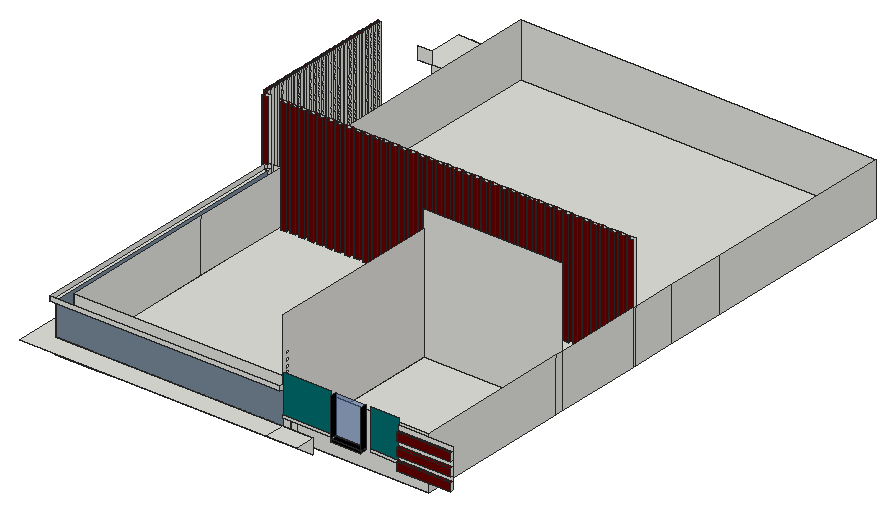
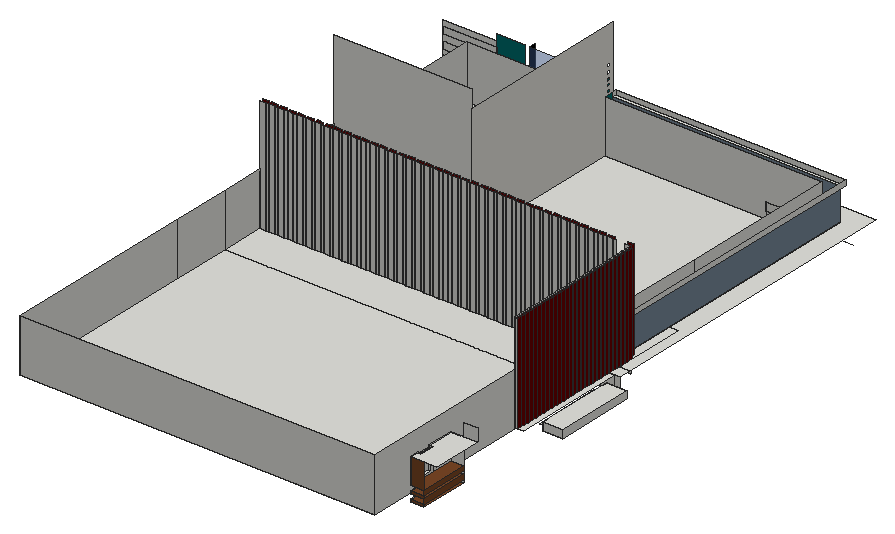
# SketchUp Ruby script. Lengths in inches.
U = 1.inch
M = Sketchup.active_model
def pt(a) = Geom::Point3d.new(a.map { |v| v * U })
def face(e, loops, mat)
  f = e.add_face(loops[0].map { |a| pt(a) })
  loops[1..].each { |l| e.add_face(l.map { |a| pt(a) }).erase! }
  f.material = f.back_material = mat if mat
  f
end
# faces: each face lists its corners as indices into pts; further lists are holes
def faces(e, pts, list, mat = nil) = list.each { |f| face(e, (f[0].is_a?(Array) ? f : [f]).map { |l| l.map { |i| pts[i] } }, mat) }
# xy, xz, yz: faces in a plane at the given z, y or x. An outline is a flat list of corners, or four numbers for a rectangle; further outlines are holes
def ring(l) = l.size == 4 ? [[l[0], l[1]], [l[2], l[1]], [l[2], l[3]], [l[0], l[3]]] : l.each_slice(2).to_a
def flat(e, list, mat, &to3) = list.each { |f| face(e, (f[0].is_a?(Array) ? f : [f]).map { |l| ring(l).map { |u, v| to3.(u, v) } }, mat) }
def xy(e, z, list, mat = nil) = flat(e, list, mat) { |x, y| [x, y, z] }
def xz(e, y, list, mat = nil) = flat(e, list, mat) { |x, z| [x, y, z] }
def yz(e, x, list, mat = nil) = flat(e, list, mat) { |y, z| [x, y, z] }
def lines(e, pts, list) = list.each { |a, b| e.add_line(pt(pts[a]), pt(pts[b])) }
# prism: a flat outline (further loops are holes) pulled along v
def prism(e, loops, v, mat = nil)
  f = face(e, loops, mat); d = Geom::Vector3d.new(v.map { |x| x * U })
  f.pushpull(f.normal.samedirection?(d) ? d.length : -d.length)
end
def box(e, o, s, mat = nil) = prism(e, [[o, [o[0] + s[0], o[1], o[2]], [o[0] + s[0], o[1] + s[1], o[2]], [o[0], o[1] + s[1], o[2]]]], [0, 0, s[2]], mat)
def at(x, y, z, deg = 0) = Geom::Transformation.translation(pt([x, y, z])) * Geom::Transformation.rotation(ORIGIN, Z_AXIS, deg.degrees)
def axes(o, x, y, z) = Geom::Transformation.new([*x, 0, *y, 0, *z, 0, *pt(o).to_a, 1])
def part(name) = M.definitions.add(name)
# library, detail: a bought-in or finely detailed component or shape, given as its bounding box
def library(name, o, s) = part(name).tap { |d| box(d.entities, o, s) }
def detail(e, o, s) = box(e.add_group.entities, o, s)
def put(e, d, t, mat = nil) = e.add_instance(d, t).tap { |i| i.material = mat if mat }
def group(e, t, mat = nil) = e.add_group.tap { |g| g.transformation = t; g.material = mat if mat }.entities
root = M.entities
M.materials.add("[0110_LightSlateGray]").color = [119, 136, 153]
M.materials.add("[Color A08]").color = [102, 0, 0]
M.materials.add("[Color H07]1").color = [0, 109, 109]
M.materials.add("[Color M09]").color = [0, 0, 0]
M.materials.add("[Marble Carrara Gold Floor Tile]").color = [225, 223, 217]
M.materials.add("[Translucent Glass Blue]1").color = [78, 117, 186]
M.materials["[Translucent Glass Blue]1"].alpha = 0.5
M.materials.add("[Wood Veneer 01]").color = [120, 70, 37]
xy(root,255.61,[[98.54,121.91,294.79,121.91,294.79,352.8,290.69,352.8,290.69,355.8,287.79,355.8,287.79,352.8,282.44,352.8,282.44,355.8,279.54,355.8,279.54,352.8,274.19,352.8,274.19,355.8,271.29,355.8,271.29,352.8,265.94,352.8,265.94,355.8,263.04,355.8,263.04,352.8,257.69,352.8,257.69,355.8,254.79,355.8,254.79,352.8,249.44,352.8,249.44,355.8,246.54,355.8,246.54,352.8,241.19,352.8,241.19,355.8,238.29,355.8,238.29,352.8,232.94,352.8,232.94,355.8,230.04,355.8,230.04,352.8,224.69,352.8,224.69,355.8,221.79,355.8,221.79,352.8,216.44,352.8,216.44,355.8,213.54,355.8,213.54,352.8,208.19,352.8,208.19,355.8,205.29,355.8,205.29,352.8,199.94,352.8,199.94,355.8,197.04,355.8,197.04,352.8,191.69,352.8,191.69,355.8,188.79,355.8,188.79,352.8,183.44,352.8,183.44,355.8,180.54,355.8,180.54,352.8,175.19,352.8,175.19,355.8,172.29,355.8,172.29,352.8,166.94,352.8,166.94,355.8,164.04,355.8,164.04,352.8,158.69,352.8,158.69,355.8,155.79,355.8,155.79,352.8,150.44,352.8,150.44,355.8,147.54,355.8,147.54,352.8,142.19,352.8,142.19,355.8,139.29,355.8,139.29,352.8,133.94,352.8,133.94,355.8,131.04,355.8,131.04,352.8,125.69,352.8,125.69,355.8,122.79,355.8,122.79,352.8,117.44,352.8,117.44,355.8,114.54,355.8,114.54,352.8,109.19,352.8,109.19,355.8,106.29,355.8,106.29,352.8,100.94,352.8,100.94,355.8,98.54,355.8],[294.79,121.91,419.79,272.1],[294.79,272.1,419.79,272.1,419.79,352.8,414.44,352.8,414.44,355.8,411.54,355.8,411.54,352.8,406.19,352.8,406.19,355.8,403.29,355.8,403.29,352.8,397.94,352.8,397.94,355.8,395.04,355.8,395.04,352.8,389.69,352.8,389.69,355.8,386.79,355.8,386.79,352.8,381.44,352.8,381.44,355.8,378.54,355.8,378.54,352.8,373.19,352.8,373.19,355.8,370.29,355.8,370.29,352.8,364.94,352.8,364.94,355.8,362.04,355.8,362.04,352.8,356.69,352.8,356.69,355.8,353.79,355.8,353.79,352.8,348.44,352.8,348.44,355.8,345.54,355.8,345.54,352.8,340.19,352.8,340.19,355.8,337.29,355.8,337.29,352.8,331.94,352.8,331.94,355.8,329.04,355.8,329.04,352.8,323.69,352.8,323.69,355.8,320.79,355.8,320.79,352.8,315.44,352.8,315.44,355.8,312.54,355.8,312.54,352.8,307.19,352.8,307.19,355.8,304.29,355.8,304.29,352.8,298.94,352.8,298.94,355.8,296.04,355.8,296.04,352.8,294.79,352.8],[100.94,352.8,106.29,355.8],[109.19,352.8,114.54,355.8],
  [117.44,352.8,122.79,355.8],[125.69,352.8,131.04,355.8],[133.94,352.8,139.29,355.8],[142.19,352.8,147.54,355.8],[150.44,352.8,155.79,355.8],
  [158.69,352.8,164.04,355.8],[166.94,352.8,172.29,355.8],[175.19,352.8,180.54,355.8],[183.44,352.8,188.79,355.8],[191.69,352.8,197.04,355.8],
  [199.94,352.8,205.29,355.8],[208.19,352.8,213.54,355.8],[216.44,352.8,221.79,355.8],[224.69,352.8,230.04,355.8],[232.94,352.8,238.29,355.8],
  [241.19,352.8,246.54,355.8],[249.44,352.8,254.79,355.8],[257.69,352.8,263.04,355.8],[265.94,352.8,271.29,355.8],[274.19,352.8,279.54,355.8],
  [282.44,352.8,287.79,355.8],[290.69,352.8,294.79,355.8],[294.79,352.8,296.04,355.8],[298.94,352.8,304.29,355.8],[307.19,352.8,312.54,355.8],
  [315.44,352.8,320.79,355.8],[323.69,352.8,329.04,355.8],[331.94,352.8,337.29,355.8],[340.19,352.8,345.54,355.8],[348.44,352.8,353.79,355.8],
  [356.69,352.8,362.04,355.8],[364.94,352.8,370.29,355.8],[373.19,352.8,378.54,355.8],[381.44,352.8,386.79,355.8],[389.69,352.8,395.04,355.8],
  [397.94,352.8,403.29,355.8],[406.19,352.8,411.54,355.8],[414.44,352.8,419.79,355.8],[98.54,355.8,419.79,396.17],[98.54,396.17,419.79,627.48]])
xy(root,256.05,[[77.54,552.74,89.54,598.37]],"[Wood Veneer 01]")
xy(root,258.45,[[77.54,552.74,89.54,598.37]],"[Wood Veneer 01]")
xy(root,260.5,[[81.04,397.54,84.04,459.54]])
xy(root,260.625,[[57.6,393.2,57.6,465.79,76.23,465.79,76.23,459.54,81.04,459.54,81.04,397.54,76.23,397.54,76.23,393.2]])
xy(root,261.93,[[121.875,112.91,149.09,121.91]])
xy(root,262.86,[[77.54,552.74,89.54,598.37]],"[Wood Veneer 01]")
xy(root,265.27,[[77.54,552.74,89.54,598.37]],"[Wood Veneer 01]")
xy(root,267.49,[[57.6,393.2,76.23,465.79]])
xy(root,269.67,[[77.54,552.74,89.54,598.37]],"[Wood Veneer 01]")
xy(root,269.74,[[72.04,94.04,294.79,94.04,294.79,112.91,89.54,112.91,89.54,305.6,80.6,305.6,80.6,372.52,72.04,372.52],[294.79,94.04,322.48,112.91],[80.6,305.6,89.54,305.6,89.54,352.8,84.44,352.8,84.44,355.8,84.04,355.8,84.04,359,81.04,359,81.04,361.77,84.04,361.77,84.04,363,81.04,363,81.04,365.77,84.04,365.77,84.04,367.5,81.04,367.5,81.04,370.27,84.04,370.27,84.04,372.0625,81.04,372.0625,81.04,374.83,84.04,374.83,84.04,376.5625,81.04,376.5625,81.04,379.33,84.04,379.33,84.04,381.0625,81.04,381.0625,81.04,383.83,84.04,383.83,84.04,383.99,72.04,383.99,72.04,372.52,80.6,372.52],[84.44,352.8,89.54,355.8],[84.04,355.8,89.54,383.99],
  [81.04,359,84.04,361.77],[81.04,363,84.04,365.77],[81.04,367.5,84.04,370.27],[81.04,372.0625,84.04,374.83],[81.04,376.5625,84.04,379.33],
  [81.04,381.0625,84.04,383.83],[76.23,383.99,84.04,383.99,84.04,385.5625,81.04,385.5625,81.04,388.33,84.04,388.33,84.04,390.0625,81.04,390.0625,81.04,392.83,84.04,392.83,84.04,394.5625,81.04,394.5625,81.04,397.33,84.04,397.33,84.04,399.0625,81.04,399.0625,81.04,401.83,84.04,401.83,84.04,403.5625,81.04,403.5625,81.04,406.33,84.04,406.33,84.04,408.0625,81.04,408.0625,81.04,410.83,84.04,410.83,84.04,412.5625,81.04,412.5625,81.04,415.33,84.04,415.33,84.04,417.0625,81.04,417.0625,81.04,419.83,84.04,419.83,84.04,421.5625,81.04,421.5625,81.04,424.33,84.04,424.33,84.04,426.0625,81.04,426.0625,81.04,428.83,84.04,428.83,84.04,430.5625,81.04,430.5625,81.04,433.33,84.04,433.33,84.04,435.0625,81.04,435.0625,81.04,437.83,84.04,437.83,84.04,439.5625,81.04,439.5625,81.04,442.33,84.04,442.33,84.04,444.0625,81.04,444.0625,81.04,446.83,84.04,446.83,84.04,448.5625,81.04,448.5625,81.04,451.33,84.04,451.33,84.04,453.0625,81.04,453.0625,81.04,455.83,84.04,455.83,84.04,457.5625,81.04,457.5625,81.04,460.33,84.04,460.33,84.04,462.0625,81.04,462.0625,81.04,464.83,84.04,464.83,84.04,466.5625,81.04,466.5625,81.04,469.33,84.04,469.33,84.04,471.0625,81.04,471.0625,81.04,473.83,84.04,473.83,84.04,475.5625,81.04,475.5625,81.04,478.33,84.04,478.33,84.04,480.0625,81.04,480.0625,81.04,482.83,84.04,482.83,84.04,484.5625,81.04,484.5625,81.04,487.33,76.23,487.33],[81.04,385.5625,84.04,388.33],[81.04,390.0625,84.04,392.83],[81.04,394.5625,84.04,397.33],
  [81.04,399.0625,84.04,401.83],[81.04,403.5625,84.04,406.33],[81.04,408.0625,83.98,410.83],[83.98,408.0625,84.04,410.83],[81.04,412.5625,84.04,415.33],
  [81.04,417.0625,84.04,419.83],[81.04,421.5625,84.04,424.33],[81.04,426.0625,84.04,428.83],[81.04,430.5625,84.04,433.33],[81.04,435.0625,84.04,437.83],
  [81.04,439.5625,84.04,442.33],[81.04,444.0625,84.04,446.83],[81.04,448.5625,84.04,451.33],[81.04,453.0625,84.04,455.83],[81.04,457.5625,84.04,460.33],
  [81.04,462.0625,84.04,464.83],[81.04,466.5625,84.04,469.33],[81.04,471.0625,84.04,473.83],[81.04,475.5625,84.04,478.33],[81.04,480.0625,84.04,482.83],
  [81.04,484.5625,84.04,487.33]])
xy(root,272.06,[[400.27,109.91,449.03,112.91]],"[Color A08]")
xy(root,272.23,[[86.54,577.37,89.54,590.18]])
xy(root,273.61,[[86.54,578.75,89.54,588.8]])
xy(root,276.34,[[343.08,106.91,369.95,112.91]],"[Color M09]")
xy(root,278.72,[[343.08,106.91,369.95,112.91]],"[Color M09]")
xy(root,278.95,[[400.27,109.91,449.03,112.91]],"[Color A08]")
xy(root,283.81,[[400.27,109.91,449.03,112.91]],"[Color A08]")
xy(root,290.7,[[400.27,109.91,449.03,112.91]],"[Color A08]")
xy(root,291.58,[[86.54,578.75,89.54,588.8]])
xy(root,292.96,[[65.54,552.74,65.54,598.37,89.54,598.37,89.54,590.18,86.54,590.18,86.54,577.37,89.54,577.37,89.54,552.74]])
xy(root,296.12,[[400.27,109.91,449.03,112.91]],"[Color A08]")
xy(root,299.34,[[86.54,109.91,86.54,352.8,89.54,352.8,89.54,112.91,294.79,112.91,294.79,109.91],[86.54,352.8,89.54,355.8]])
xy(root,303.01,[[400.27,109.91,449.03,112.91]],"[Color A08]")
xz(root,106.91,[[343.08,276.34,369.95,278.72]],"[Color M09]")
xz(root,109.91,[[86.54,299.34,294.79,303.61]])
xz(root,109.91,[[400.27,272.06,449.03,278.95],[400.27,283.81,449.03,290.7],[400.27,296.12,449.03,303.01]],"[Color A08]")
xz(root,112.91,[[89.54,255.61,121.875,269.74],[121.875,255.61,149.09,261.93],[149.09,255.61,294.79,269.74],[294.79,255.61,322.48,269.74],[121.875,261.93,149.09,269.74],
  [400.27,272.06,449.03,278.95],[294.79,276.34,338.5625,278.72],[343.08,276.34,369.95,278.72],[374.46,276.34,400.27,278.72],[400.27,278.95,449.03,283.81],
  [400.27,283.81,449.03,290.7],[400.27,290.7,449.03,296.12],[400.27,296.12,449.03,303.01],[400.27,303.01,449.03,307.31]])
xz(root,112.91,[[89.54,269.74,294.79,299.34]],"[0110_LightSlateGray]")
xz(root,112.91,[[294.79,278.72,338.5625,313.34],[374.46,278.72,400.27,313.34]],"[Color H07]1")
xz(root,112.91,[[343.08,278.72,369.95,313.34]],"[Translucent Glass Blue]1")
xz(root,121.91,[[98.54,255.61,98.54,303.61,294.79,303.61,294.79,255.61,149.09,255.61,149.09,269.74,121.875,269.74,121.875,255.61],[121.875,255.61,149.09,261.93],[294.79,255.61,300.79,303.61],[300.79,255.61,419.79,303.61],[121.875,261.93,149.09,269.74]])
xz(root,272.1,[[294.79,255.61,419.79,375.61]])
xz(root,352.8,[[100.94,255.61,106.29,359.2],[109.19,255.61,114.54,359.2],[117.44,255.61,122.79,359.2],[125.69,255.61,131.04,359.2],[133.94,255.61,139.29,359.2],
  [142.19,255.61,147.54,359.2],[150.44,255.61,155.79,359.2],[158.69,255.61,164.04,359.2],[166.94,255.61,172.29,359.2],[175.19,255.61,180.54,359.2],
  [183.44,255.61,188.79,359.2],[191.69,255.61,197.04,359.2],[199.94,255.61,205.29,359.2],[208.19,255.61,213.54,359.2],[216.44,255.61,221.79,359.2],
  [224.69,255.61,230.04,359.2],[232.94,255.61,238.29,359.2],[241.19,255.61,246.54,359.2],[249.44,255.61,254.79,359.2],[257.69,255.61,263.04,359.2],
  [265.94,255.61,271.29,359.2],[274.19,255.61,279.54,359.2],[282.44,255.61,287.79,359.2],[290.69,255.61,296.04,359.2],[298.94,255.61,304.29,359.2],
  [307.19,255.61,312.54,359.2],[315.44,255.61,320.79,359.2],[323.69,255.61,329.04,359.2],[331.94,255.61,337.29,359.2],[340.19,255.61,345.54,359.2],
  [348.44,255.61,353.79,359.2],[356.69,255.61,362.04,359.2],[364.94,255.61,370.29,359.2],[373.19,255.61,378.54,359.2],[381.44,255.61,386.79,359.2],
  [389.69,255.61,395.04,359.2],[397.94,255.61,403.29,359.2],[406.19,255.61,411.54,359.2],[414.44,255.61,419.79,359.2],[84.44,269.74,89.54,269.74,89.54,299.34,86.54,299.34,86.54,303.61,89.79,303.61,89.79,359.2,84.44,359.2]],"[Color A08]")
xz(root,355.8,[[84.44,255.61,89.79,255.61,89.79,303.61,89.54,303.61,89.54,269.74,84.44,269.74],[92.69,255.61,98.04,303.61],[98.54,255.61,100.94,255.61,100.94,359.2,98.04,359.2,98.04,303.61,98.54,303.61],[100.94,255.61,106.29,359.2],[106.29,255.61,109.19,359.2],
  [109.19,255.61,114.54,359.2],[114.54,255.61,117.44,359.2],[117.44,255.61,122.79,359.2],[122.79,255.61,125.69,359.2],[125.69,255.61,131.04,359.2],
  [131.04,255.61,133.94,359.2],[133.94,255.61,139.29,359.2],[139.29,255.61,142.19,359.2],[142.19,255.61,147.54,359.2],[147.54,255.61,150.44,359.2],
  [150.44,255.61,155.79,359.2],[155.79,255.61,158.69,359.2],[158.69,255.61,164.04,359.2],[164.04,255.61,166.94,359.2],[166.94,255.61,172.29,359.2],
  [172.29,255.61,175.19,359.2],[175.19,255.61,180.54,359.2],[180.54,255.61,183.44,359.2],[183.44,255.61,188.79,359.2],[188.79,255.61,191.69,359.2],
  [191.69,255.61,197.04,359.2],[197.04,255.61,199.94,359.2],[199.94,255.61,205.29,359.2],[205.29,255.61,208.19,359.2],[208.19,255.61,213.54,359.2],
  [213.54,255.61,216.44,359.2],[216.44,255.61,221.79,359.2],[221.79,255.61,224.69,359.2],[224.69,255.61,230.04,359.2],[230.04,255.61,232.94,359.2],
  [232.94,255.61,238.29,359.2],[238.29,255.61,241.19,359.2],[241.19,255.61,246.54,359.2],[246.54,255.61,249.44,359.2],[249.44,255.61,254.79,359.2],
  [254.79,255.61,257.69,359.2],[257.69,255.61,263.04,359.2],[263.04,255.61,265.94,359.2],[265.94,255.61,271.29,359.2],[271.29,255.61,274.19,359.2],
  [274.19,255.61,279.54,359.2],[279.54,255.61,282.44,359.2],[282.44,255.61,287.79,359.2],[287.79,255.61,290.69,359.2],[290.69,255.61,296.04,359.2],
  [296.04,255.61,298.94,359.2],[298.94,255.61,304.29,359.2],[304.29,255.61,307.19,359.2],[307.19,255.61,312.54,359.2],[312.54,255.61,315.44,359.2],
  [315.44,255.61,320.79,359.2],[320.79,255.61,323.69,359.2],[323.69,255.61,329.04,359.2],[329.04,255.61,331.94,359.2],[331.94,255.61,337.29,359.2],
  [337.29,255.61,340.19,359.2],[340.19,255.61,345.54,359.2],[345.54,255.61,348.44,359.2],[348.44,255.61,353.79,359.2],[353.79,255.61,356.69,359.2],
  [356.69,255.61,362.04,359.2],[362.04,255.61,364.94,359.2],[364.94,255.61,370.29,359.2],[370.29,255.61,373.19,359.2],[373.19,255.61,378.54,359.2],
  [378.54,255.61,381.44,359.2],[381.44,255.61,386.79,359.2],[386.79,255.61,389.69,359.2],[389.69,255.61,395.04,359.2],[395.04,255.61,397.94,359.2],
  [397.94,255.61,403.29,359.2],[403.29,255.61,406.19,359.2],[406.19,255.61,411.54,359.2],[411.54,255.61,414.44,359.2],[414.44,255.61,419.79,359.2],
  [84.44,269.74,84.44,359.2,89.79,359.2,89.79,303.61,86.54,303.61,86.54,299.34,89.54,299.34,89.54,269.74],[86.54,299.34,89.54,303.61]])
xz(root,355.8,[[84.04,269.74,84.44,359.2]],"[Color A08]")
xz(root,359,[[81.04,269.74,84.04,359.2]],"[Color A08]")
xz(root,361.77,[[81.04,269.74,84.04,359.2]],"[Color A08]")
xz(root,363,[[81.04,269.74,84.04,359.2]],"[Color A08]")
xz(root,365.77,[[81.04,269.74,84.04,359.2]],"[Color A08]")
xz(root,367.5,[[81.04,269.74,84.04,359.2]],"[Color A08]")
xz(root,370.27,[[81.04,269.74,84.04,359.2]],"[Color A08]")
xz(root,372.0625,[[81.04,269.74,84.04,359.2]],"[Color A08]")
xz(root,374.83,[[81.04,269.74,84.04,359.2]],"[Color A08]")
xz(root,376.5625,[[81.04,269.74,84.04,359.2]],"[Color A08]")
xz(root,379.33,[[81.04,269.74,84.04,359.2]],"[Color A08]")
xz(root,381.0625,[[81.04,269.74,84.04,359.2]],"[Color A08]")
xz(root,383.83,[[81.04,269.74,84.04,359.2]],"[Color A08]")
xz(root,383.99,[[72.04,255.61,76.23,269.74],[76.23,255.61,89.54,269.74]])
xz(root,385.5625,[[81.04,269.74,84.04,359.2]],"[Color A08]")
xz(root,388.33,[[81.04,269.74,84.04,359.2]],"[Color A08]")
xz(root,390.0625,[[81.04,269.74,84.04,359.2]],"[Color A08]")
xz(root,392.83,[[81.04,269.74,84.04,359.2]],"[Color A08]")
xz(root,393.2,[[57.6,260.625,76.23,267.49]])
xz(root,394.5625,[[81.04,269.74,84.04,359.2]],"[Color A08]")
xz(root,397.33,[[81.04,269.74,84.04,359.2]],"[Color A08]")
xz(root,399.0625,[[81.04,269.74,84.04,359.2]],"[Color A08]")
xz(root,401.83,[[81.04,269.74,84.04,359.2]],"[Color A08]")
xz(root,403.5625,[[81.04,269.74,84.04,359.2]],"[Color A08]")
xz(root,406.33,[[81.04,269.74,84.04,359.2]],"[Color A08]")
xz(root,408.0625,[[83.98,269.74,84.04,359.2]])
xz(root,408.0625,[[81.04,269.74,83.98,359.2]],"[Color A08]")
xz(root,410.83,[[83.98,269.74,84.04,359.2]])
xz(root,410.83,[[81.04,269.74,83.98,359.2]],"[Color A08]")
xz(root,412.5625,[[81.04,269.74,84.04,359.2]],"[Color A08]")
xz(root,415.33,[[81.04,269.74,84.04,359.2]],"[Color A08]")
xz(root,417.0625,[[81.04,269.74,84.04,359.2]],"[Color A08]")
xz(root,419.83,[[81.04,269.74,84.04,359.2]],"[Color A08]")
xz(root,421.5625,[[81.04,269.74,84.04,359.2]],"[Color A08]")
xz(root,424.33,[[81.04,269.74,84.04,359.2]],"[Color A08]")
xz(root,426.0625,[[81.04,269.74,84.04,359.2]],"[Color A08]")
xz(root,428.83,[[81.04,269.74,84.04,359.2]],"[Color A08]")
xz(root,430.5625,[[81.04,269.74,84.04,359.2]],"[Color A08]")
xz(root,433.33,[[81.04,269.74,84.04,359.2]],"[Color A08]")
xz(root,435.0625,[[81.04,269.74,84.04,359.2]],"[Color A08]")
xz(root,437.83,[[81.04,269.74,84.04,359.2]],"[Color A08]")
xz(root,439.5625,[[81.04,269.74,84.04,359.2]],"[Color A08]")
xz(root,442.33,[[81.04,269.74,84.04,359.2]],"[Color A08]")
xz(root,444.0625,[[81.04,269.74,84.04,359.2]],"[Color A08]")
xz(root,446.83,[[81.04,269.74,84.04,359.2]],"[Color A08]")
xz(root,448.5625,[[81.04,269.74,84.04,359.2]],"[Color A08]")
xz(root,451.33,[[81.04,269.74,84.04,359.2]],"[Color A08]")
xz(root,453.0625,[[81.04,269.74,84.04,359.2]],"[Color A08]")
xz(root,455.83,[[81.04,269.74,84.04,359.2]],"[Color A08]")
xz(root,457.5625,[[81.04,269.74,84.04,359.2]],"[Color A08]")
xz(root,460.33,[[81.04,269.74,84.04,359.2]],"[Color A08]")
xz(root,462.0625,[[81.04,269.74,84.04,359.2]],"[Color A08]")
xz(root,464.83,[[81.04,269.74,84.04,359.2]],"[Color A08]")
xz(root,465.79,[[57.6,260.625,76.23,267.49]])
xz(root,466.5625,[[81.04,269.74,84.04,359.2]],"[Color A08]")
xz(root,469.33,[[81.04,269.74,84.04,359.2]],"[Color A08]")
xz(root,471.0625,[[81.04,269.74,84.04,359.2]],"[Color A08]")
xz(root,473.83,[[81.04,269.74,84.04,359.2]],"[Color A08]")
xz(root,475.5625,[[81.04,269.74,84.04,359.2]],"[Color A08]")
xz(root,478.33,[[81.04,269.74,84.04,359.2]],"[Color A08]")
xz(root,480.0625,[[81.04,269.74,84.04,359.2]],"[Color A08]")
xz(root,482.83,[[81.04,269.74,84.04,359.2]],"[Color A08]")
xz(root,484.5625,[[81.04,269.74,84.04,359.2]],"[Color A08]")
xz(root,487.33,[[81.04,269.74,84.04,359.2]])
xz(root,552.74,[[77.54,256.05,89.54,258.45],[77.54,262.86,89.54,265.27],[77.54,269.67,89.54,292.96],[65.54,292.96,77.54,304.46]])
xz(root,577.37,[[86.54,272.23,89.54,292.96]])
xz(root,578.75,[[86.54,273.61,89.54,291.58]])
xz(root,588.8,[[86.54,273.61,89.54,291.58]])
xz(root,590.18,[[86.54,272.23,89.54,292.96]])
xz(root,598.37,[[77.54,256.05,89.54,258.45],[77.54,262.86,89.54,265.27],[77.54,269.67,89.54,292.96]],"[Wood Veneer 01]")
xz(root,627.48,[[98.54,255.61,419.79,303.61]])
yz(root,57.6,[[393.2,260.625,465.79,267.49]])
yz(root,76.23,[[393.2,260.625,396.51,267.49],[459.54,260.625,465.79,267.49]])
yz(root,77.54,[[552.74,258.45,598.37,262.86],[552.74,265.27,598.37,269.67]],"[Wood Veneer 01]")
yz(root,81.04,[[397.54,260.5,459.54,260.625]])
yz(root,81.04,[[359,269.74,361.77,359.2],[363,269.74,365.77,359.2],[367.5,269.74,370.27,359.2],[372.0625,269.74,374.83,359.2],[376.5625,269.74,379.33,359.2],
  [381.0625,269.74,383.83,359.2],[385.5625,269.74,388.33,359.2],[390.0625,269.74,392.83,359.2],[394.5625,269.74,397.33,359.2],[399.0625,269.74,401.83,359.2],
  [403.5625,269.74,406.33,359.2],[408.0625,269.74,410.83,359.2],[412.5625,269.74,415.33,359.2],[417.0625,269.74,419.83,359.2],[421.5625,269.74,424.33,359.2],
  [426.0625,269.74,428.83,359.2],[430.5625,269.74,433.33,359.2],[435.0625,269.74,437.83,359.2],[439.5625,269.74,442.33,359.2],[444.0625,269.74,446.83,359.2],
  [448.5625,269.74,451.33,359.2],[453.0625,269.74,455.83,359.2],[457.5625,269.74,460.33,359.2],[462.0625,269.74,464.83,359.2],[466.5625,269.74,469.33,359.2],
  [471.0625,269.74,473.83,359.2],[475.5625,269.74,478.33,359.2],[480.0625,269.74,482.83,359.2],[484.5625,269.74,487.33,359.2]],"[Color A08]")
yz(root,83.98,[[408.0625,269.74,410.83,359.2]])
yz(root,84.04,[[359,269.74,361.77,359.2],[361.77,269.74,363,359.2],[363,269.74,365.77,359.2],[365.77,269.74,367.5,359.2],[367.5,269.74,370.27,359.2],
  [370.27,269.74,372.0625,359.2],[372.0625,269.74,374.83,359.2],[374.83,269.74,376.5625,359.2],[376.5625,269.74,379.33,359.2],[379.33,269.74,381.0625,359.2],
  [381.0625,269.74,383.83,359.2],[383.83,269.74,385.5625,359.2],[385.5625,269.74,388.33,359.2],[388.33,269.74,390.0625,359.2],[390.0625,269.74,392.83,359.2],
  [392.83,269.74,394.5625,359.2],[394.5625,269.74,397.33,359.2],[397.33,269.74,399.0625,359.2],[399.0625,269.74,401.83,359.2],[401.83,269.74,403.5625,359.2],
  [403.5625,269.74,406.33,359.2],[406.33,269.74,408.0625,359.2],[408.0625,269.74,410.83,359.2],[410.83,269.74,412.5625,359.2],[412.5625,269.74,415.33,359.2],
  [415.33,269.74,417.0625,359.2],[417.0625,269.74,419.83,359.2],[419.83,269.74,421.5625,359.2],[421.5625,269.74,424.33,359.2],[424.33,269.74,426.0625,359.2],
  [426.0625,269.74,428.83,359.2],[428.83,269.74,430.5625,359.2],[430.5625,269.74,433.33,359.2],[433.33,269.74,435.0625,359.2],[435.0625,269.74,437.83,359.2],
  [437.83,269.74,439.5625,359.2],[439.5625,269.74,442.33,359.2],[442.33,269.74,444.0625,359.2],[444.0625,269.74,446.83,359.2],[446.83,269.74,448.5625,359.2],
  [448.5625,269.74,451.33,359.2],[451.33,269.74,453.0625,359.2],[453.0625,269.74,455.83,359.2],[455.83,269.74,457.5625,359.2],[457.5625,269.74,460.33,359.2],
  [460.33,269.74,462.0625,359.2],[462.0625,269.74,464.83,359.2],[464.83,269.74,466.5625,359.2],[466.5625,269.74,469.33,359.2],[469.33,269.74,471.0625,359.2],
  [471.0625,269.74,473.83,359.2],[473.83,269.74,475.5625,359.2],[475.5625,269.74,478.33,359.2],[478.33,269.74,480.0625,359.2],[480.0625,269.74,482.83,359.2],
  [482.83,269.74,484.5625,359.2],[484.5625,269.74,487.33,359.2]])
yz(root,84.04,[[355.8,269.74,359,359.2]],"[Color A08]")
yz(root,84.44,[[352.8,269.74,355.8,359.2]],"[Color A08]")
yz(root,86.54,[[[577.37,272.23,590.18,292.96],[578.75,273.61,588.8,291.58]],[109.91,299.34,352.8,303.61],[352.8,299.34,355.8,303.61]])
yz(root,89.54,[[112.91,255.61,305.6,269.74],[305.6,255.61,383.99,269.74],[552.74,256.05,598.37,258.45],[552.74,262.86,598.37,265.27],[552.74,269.67,552.74,292.96,577.37,292.96,577.37,272.23,590.18,272.23,590.18,292.96,598.37,292.96,598.37,269.67],
  [352.8,269.74,355.8,299.34],[578.75,273.61,588.8,291.58]])
yz(root,89.54,[[112.91,269.74,352.8,299.34]],"[0110_LightSlateGray]")
yz(root,98.54,[[121.91,255.61,266.1,303.61],[266.1,255.61,355.8,303.61],[355.8,255.61,396.17,303.61],[396.17,255.61,627.48,303.61]])
yz(root,100.94,[[352.8,255.61,355.8,359.2]],"[Color A08]")
yz(root,106.29,[[352.8,255.61,355.8,359.2]],"[Color A08]")
yz(root,109.19,[[352.8,255.61,355.8,359.2]],"[Color A08]")
yz(root,114.54,[[352.8,255.61,355.8,359.2]],"[Color A08]")
yz(root,117.44,[[352.8,255.61,355.8,359.2]],"[Color A08]")
yz(root,121.875,[[112.91,261.93,121.91,269.74]])
yz(root,122.79,[[352.8,255.61,355.8,359.2]],"[Color A08]")
yz(root,125.69,[[352.8,255.61,355.8,359.2]],"[Color A08]")
yz(root,131.04,[[352.8,255.61,355.8,359.2]],"[Color A08]")
yz(root,133.94,[[352.8,255.61,355.8,359.2]],"[Color A08]")
yz(root,139.29,[[352.8,255.61,355.8,359.2]],"[Color A08]")
yz(root,142.19,[[352.8,255.61,355.8,359.2]],"[Color A08]")
yz(root,147.54,[[352.8,255.61,355.8,359.2]],"[Color A08]")
yz(root,149.09,[[112.91,261.93,121.91,269.74]])
yz(root,150.44,[[352.8,255.61,355.8,359.2]],"[Color A08]")
yz(root,155.79,[[352.8,255.61,355.8,359.2]],"[Color A08]")
yz(root,158.69,[[352.8,255.61,355.8,359.2]],"[Color A08]")
yz(root,164.04,[[352.8,255.61,355.8,359.2]],"[Color A08]")
yz(root,166.94,[[352.8,255.61,355.8,359.2]],"[Color A08]")
yz(root,172.29,[[352.8,255.61,355.8,359.2]],"[Color A08]")
yz(root,175.19,[[352.8,255.61,355.8,359.2]],"[Color A08]")
yz(root,180.54,[[352.8,255.61,355.8,359.2]],"[Color A08]")
yz(root,183.44,[[352.8,255.61,355.8,359.2]],"[Color A08]")
yz(root,188.79,[[352.8,255.61,355.8,359.2]],"[Color A08]")
yz(root,191.69,[[352.8,255.61,355.8,359.2]],"[Color A08]")
yz(root,197.04,[[352.8,255.61,355.8,359.2]],"[Color A08]")
yz(root,199.94,[[352.8,255.61,355.8,359.2]],"[Color A08]")
yz(root,205.29,[[352.8,255.61,355.8,359.2]],"[Color A08]")
yz(root,208.19,[[352.8,255.61,355.8,359.2]],"[Color A08]")
yz(root,213.54,[[352.8,255.61,355.8,359.2]],"[Color A08]")
yz(root,216.44,[[352.8,255.61,355.8,359.2]],"[Color A08]")
yz(root,221.79,[[352.8,255.61,355.8,359.2]],"[Color A08]")
yz(root,224.69,[[352.8,255.61,355.8,359.2]],"[Color A08]")
yz(root,230.04,[[352.8,255.61,355.8,359.2]],"[Color A08]")
yz(root,232.94,[[352.8,255.61,355.8,359.2]],"[Color A08]")
yz(root,238.29,[[352.8,255.61,355.8,359.2]],"[Color A08]")
yz(root,241.19,[[352.8,255.61,355.8,359.2]],"[Color A08]")
yz(root,246.54,[[352.8,255.61,355.8,359.2]],"[Color A08]")
yz(root,249.44,[[352.8,255.61,355.8,359.2]],"[Color A08]")
yz(root,254.79,[[352.8,255.61,355.8,359.2]],"[Color A08]")
yz(root,257.69,[[352.8,255.61,355.8,359.2]],"[Color A08]")
yz(root,263.04,[[352.8,255.61,355.8,359.2]],"[Color A08]")
yz(root,265.94,[[352.8,255.61,355.8,359.2]],"[Color A08]")
yz(root,271.29,[[352.8,255.61,355.8,359.2]],"[Color A08]")
yz(root,274.19,[[352.8,255.61,355.8,359.2]],"[Color A08]")
yz(root,279.54,[[352.8,255.61,355.8,359.2]],"[Color A08]")
yz(root,282.44,[[352.8,255.61,355.8,359.2]],"[Color A08]")
yz(root,287.79,[[352.8,255.61,355.8,359.2]],"[Color A08]")
yz(root,290.69,[[352.8,255.61,355.8,359.2]],"[Color A08]")
yz(root,294.79,[[109.91,299.34,112.91,303.61]])
yz(root,294.79,[[[121.91,255.61,121.91,303.61,112.91,303.61,112.91,359.87,272.1,359.87,272.1,255.61],[118.2,325.72,118.65,325.77,119.08,325.95,119.4375,326.23,119.72,326.59,119.89,327.01,119.95,327.47,119.89,327.92,119.72,328.34,119.4375,328.7,119.08,328.98,118.65,329.16,118.2,329.22,117.75,329.16,117.33,328.98,116.96,328.7,116.6875,328.34,116.51,327.92,116.45,327.47,116.51,327.01,116.6875,326.59,116.96,326.23,117.33,325.95,117.75,325.77],[118.2,319.59,118.65,319.65,119.08,319.82,119.4375,320.1,119.72,320.47,119.89,320.89,119.95,321.34,119.89,321.79,119.72,322.22,119.4375,322.58,119.08,322.86,118.65,323.03,118.2,323.09,117.75,323.03,117.33,322.86,116.96,322.58,116.6875,322.22,116.51,321.79,116.45,321.34,116.51,320.89,116.6875,320.47,116.96,320.1,117.33,319.82,117.75,319.65],[118.2,314.15,118.65,314.21,119.08,314.39,119.4375,314.67,119.72,315.03,119.89,315.45,119.95,315.9,119.89,316.36,119.72,316.78,119.4375,317.14,119.08,317.42,118.65,317.59,118.2,317.65,117.75,317.59,117.33,317.42,116.96,317.14,116.6875,316.78,116.51,316.36,116.45,315.9,116.51,315.45,116.6875,315.03,116.96,314.67,117.33,314.39,117.75,314.21],[118.2,309.59,118.65,309.65,119.08,309.82,119.4375,310.1,119.72,310.47,119.89,310.89,119.95,311.34,119.89,311.79,119.72,312.22,119.4375,312.58,119.08,312.86,118.65,313.03,118.2,313.09,117.75,313.03,117.33,312.86,116.96,312.58,116.6875,312.22,116.51,311.79,116.45,311.34,116.51,310.89,116.6875,310.47,116.96,310.1,117.33,309.82,117.75,309.65],[118.2,304.65,118.65,304.71,119.08,304.89,119.4375,305.17,119.72,305.53,119.89,305.95,119.95,306.4,119.89,306.86,119.72,307.28,119.4375,307.64,119.08,307.92,118.65,308.09,118.2,308.15,117.75,308.09,117.33,307.92,116.96,307.64,116.6875,307.28,116.51,306.86,116.45,306.4,116.51,305.95,116.6875,305.53,116.96,305.17,117.33,304.89,117.75,304.71]]],"[Marble Carrara Gold Floor Tile]")
yz(root,296.04,[[352.8,255.61,355.8,359.2]],"[Color A08]")
yz(root,298.94,[[352.8,255.61,355.8,359.2]],"[Color A08]")
yz(root,304.29,[[352.8,255.61,355.8,359.2]],"[Color A08]")
yz(root,307.19,[[352.8,255.61,355.8,359.2]],"[Color A08]")
yz(root,312.54,[[352.8,255.61,355.8,359.2]],"[Color A08]")
yz(root,315.44,[[352.8,255.61,355.8,359.2]],"[Color A08]")
yz(root,320.79,[[352.8,255.61,355.8,359.2]],"[Color A08]")
yz(root,323.69,[[352.8,255.61,355.8,359.2]],"[Color A08]")
yz(root,329.04,[[352.8,255.61,355.8,359.2]],"[Color A08]")
yz(root,331.94,[[352.8,255.61,355.8,359.2]],"[Color A08]")
yz(root,337.29,[[352.8,255.61,355.8,359.2]],"[Color A08]")
yz(root,340.19,[[352.8,255.61,355.8,359.2]],"[Color A08]")
yz(root,343.08,[[106.91,276.34,112.91,278.72]])
yz(root,343.08,[[106.91,278.72,112.91,313.34]],"[Color M09]")
yz(root,345.54,[[352.8,255.61,355.8,359.2]],"[Color A08]")
yz(root,348.44,[[352.8,255.61,355.8,359.2]],"[Color A08]")
yz(root,353.79,[[352.8,255.61,355.8,359.2]],"[Color A08]")
yz(root,356.69,[[352.8,255.61,355.8,359.2]],"[Color A08]")
yz(root,362.04,[[352.8,255.61,355.8,359.2]],"[Color A08]")
yz(root,364.94,[[352.8,255.61,355.8,359.2]],"[Color A08]")
yz(root,369.95,[[106.91,278.72,112.91,313.34]],"[Color M09]")
yz(root,370.29,[[352.8,255.61,355.8,359.2]],"[Color A08]")
yz(root,373.19,[[352.8,255.61,355.8,359.2]],"[Color A08]")
yz(root,378.54,[[352.8,255.61,355.8,359.2]],"[Color A08]")
yz(root,381.44,[[352.8,255.61,355.8,359.2]],"[Color A08]")
yz(root,386.79,[[352.8,255.61,355.8,359.2]],"[Color A08]")
yz(root,389.69,[[352.8,255.61,355.8,359.2]],"[Color A08]")
yz(root,395.04,[[352.8,255.61,355.8,359.2]],"[Color A08]")
yz(root,397.94,[[352.8,255.61,355.8,359.2]],"[Color A08]")
yz(root,400.27,[[109.91,272.06,112.91,276.34],[109.91,276.34,112.91,278.72],[109.91,278.72,112.91,278.95],[109.91,283.81,112.91,290.7],[109.91,296.12,112.91,303.01]],"[Color A08]")
yz(root,403.29,[[352.8,255.61,355.8,359.2]],"[Color A08]")
yz(root,406.19,[[352.8,255.61,355.8,359.2]],"[Color A08]")
yz(root,411.54,[[352.8,255.61,355.8,359.2]],"[Color A08]")
yz(root,414.44,[[352.8,255.61,355.8,359.2]],"[Color A08]")
yz(root,419.79,[[121.91,255.61,266.1,303.61],[266.1,255.61,272.1,303.61],[272.1,255.61,352.8,303.61],[352.8,255.61,355.8,303.61],[355.8,255.61,396.17,303.61],
  [396.17,255.61,449.91,303.61],[449.91,255.61,627.48,303.61]])
yz(root,449.03,[[109.91,272.06,112.91,278.95],[109.91,283.81,112.91,290.7],[109.91,296.12,112.91,303.01]])
p = [[89.54,112.91,255.61],[77.54,112.91,255.61]]
lines(root,p,[[0,1]])
